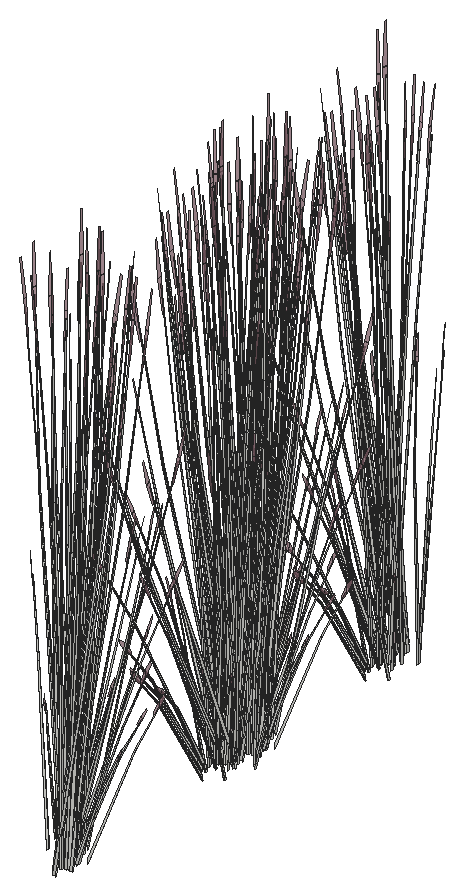
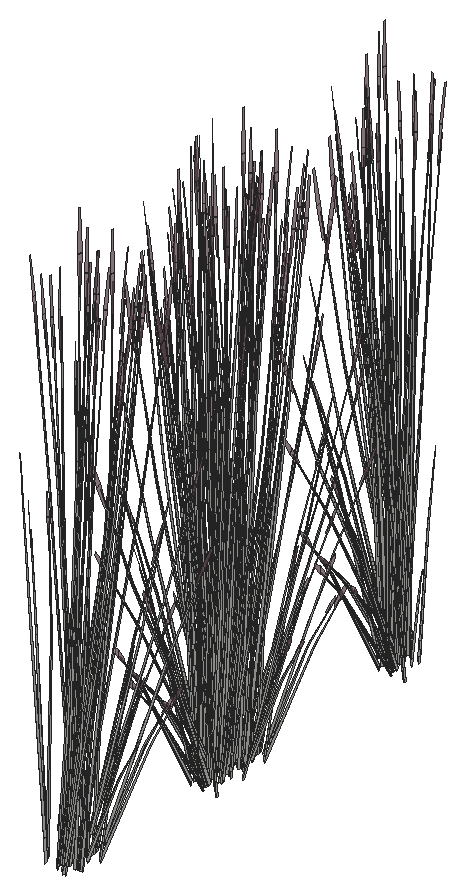
# SketchUp Ruby script. Lengths in inches.
U = 1.inch
M = Sketchup.active_model
def pt(a) = Geom::Point3d.new(a.map { |v| v * U })
def face(e, loops, mat)
  f = e.add_face(loops[0].map { |a| pt(a) })
  loops[1..].each { |l| e.add_face(l.map { |a| pt(a) }).erase! }
  f.material = f.back_material = mat if mat
  f
end
# faces: each face lists its corners as indices into pts; further lists are holes
def faces(e, pts, list, mat = nil) = list.each { |f| face(e, (f[0].is_a?(Array) ? f : [f]).map { |l| l.map { |i| pts[i] } }, mat) }
# xy, xz, yz: faces in a plane at the given z, y or x. An outline is a flat list of corners, or four numbers for a rectangle; further outlines are holes
def ring(l) = l.size == 4 ? [[l[0], l[1]], [l[2], l[1]], [l[2], l[3]], [l[0], l[3]]] : l.each_slice(2).to_a
def flat(e, list, mat, &to3) = list.each { |f| face(e, (f[0].is_a?(Array) ? f : [f]).map { |l| ring(l).map { |u, v| to3.(u, v) } }, mat) }
def xy(e, z, list, mat = nil) = flat(e, list, mat) { |x, y| [x, y, z] }
def xz(e, y, list, mat = nil) = flat(e, list, mat) { |x, z| [x, y, z] }
def yz(e, x, list, mat = nil) = flat(e, list, mat) { |y, z| [x, y, z] }
def lines(e, pts, list) = list.each { |a, b| e.add_line(pt(pts[a]), pt(pts[b])) }
# prism: a flat outline (further loops are holes) pulled along v
def prism(e, loops, v, mat = nil)
  f = face(e, loops, mat); d = Geom::Vector3d.new(v.map { |x| x * U })
  f.pushpull(f.normal.samedirection?(d) ? d.length : -d.length)
end
def box(e, o, s, mat = nil) = prism(e, [[o, [o[0] + s[0], o[1], o[2]], [o[0] + s[0], o[1] + s[1], o[2]], [o[0], o[1] + s[1], o[2]]]], [0, 0, s[2]], mat)
def at(x, y, z, deg = 0) = Geom::Transformation.translation(pt([x, y, z])) * Geom::Transformation.rotation(ORIGIN, Z_AXIS, deg.degrees)
def axes(o, x, y, z) = Geom::Transformation.new([*x, 0, *y, 0, *z, 0, *pt(o).to_a, 1])
def part(name) = M.definitions.add(name)
# library, detail: a bought-in or finely detailed component or shape, given as its bounding box
def library(name, o, s) = part(name).tap { |d| box(d.entities, o, s) }
def detail(e, o, s) = box(e.add_group.entities, o, s)
def put(e, d, t, mat = nil) = e.add_instance(d, t).tap { |i| i.material = mat if mat }
def group(e, t, mat = nil) = e.add_group.tap { |g| g.transformation = t; g.material = mat if mat }.entities
root = M.entities
M.materials.add("LightPink_Translucent").color = [144, 107, 117]
M.materials["LightPink_Translucent"].alpha = 0.75
c1 = part("blade")
p = [[2.15,0.21,22],[0,0.17,0],[0.09,0.45,0],[2.18,0.31,22],[2.29,0.31,22],[0.38,0.45,0],
  [2.48,0.24,33],[2.49,0.24,33],[2.48,0.22,33]]
faces(c1.entities,p,[[0,1,2,3],[4,5,2,3],[6,3,4,7],[8,0,3,6]])
c2 = part("seeds")
p = [[0.3,-0.1,1.38],[-0.01,-0.03,1.59],[-0.01,-0.03,0.03],[0.14,-0.07,-0.07],[0.29,-0.03,3],[0.15,0.01,3.11]]
faces(c2.entities,p,[[0,1,2,3],[1,0,4,5]],"LightPink_Translucent")
c3 = part("blade with seeds")
put(c3.entities,c1,at(0,0,0))
put(c3.entities,c2,axes([2.4,0.25,30.99],[1.5799,-0.05474,1.17369],[-0.12525,1.92788,0.29478],[-0.07173,-0.02425,1.56792]))
put(root,c3,axes([252.5625,62.65,0.99],[-0.2011,-0.44539,0.12804],[0.20266,-0.432,0.25465],[-0.02221,0.09096,1.1642]))
put(root,c3,axes([252.1875,61.98,0.6875],[0.26625,0.10025,-0.45255],[-0.05619,0.61836,-0.11877],[0.07946,0.07493,0.99892]))
put(root,c3,axes([253.36,63.06,1.2],[-0.15814,0.10094,0.83364],[0.07444,-0.41719,0.6125],[0.0839,0.02855,0.18362]))
put(root,c3,axes([251.67,64.27,0.79],[-0.25804,-0.27452,0],[0.12419,-0.5704,0],[0,0,1.1809]))
put(root,c3,axes([251.89,63.54,0.98],[-0.24993,-0.49214,-0.18284],[0.21031,-0.55263,0.40012],[-0.0673,0.05757,1.22088]))
put(root,c3,axes([251.23,64.48,0.99],[0.23955,0.30573,0.36036],[-0.14318,0.54821,0],[-0.05456,-0.06963,1.14313]))
put(root,c3,axes([252.07,62.36,1.17],[0.12419,-0.55096,0.32471],[0.25804,0.26516,-0.15627],[0,0.12701,1.04254]))
put(root,c3,axes([252.03,62.68,0.86],[0,0.70714,-0.04091],[-0.32006,0,0],[0,0.02222,1.30182]))
put(root,c3,axes([252.05,62.18,0.8],[0.15376,0.51322,-0.32471],[-0.2329,0.3614,0.15627],[0.04976,0.0635,1.04254]))
put(root,c3,axes([251.09,64.8,0.91],[-0.16003,0.61271,0],[-0.26773,-0.34169,-0.37456],[-0.06098,-0.07782,1.18819]))
put(root,c3,axes([252.73,62.67,0.99],[0,-0.61145,0.36036],[0.28637,0,0],[0,0.13926,1.14313]))
put(root,c3,axes([252.01,63.13,1.17],[0.27795,-0.03775,0.32471],[0.02514,0.62656,-0.15627],[-0.04976,0.0635,1.04254]))
put(root,c3,axes([252.18,62.49,1.09],[0.23848,-0.17832,0.10509],[0.08351,0.5092,-0.30009],[0,0.11207,0.91989]))
put(root,c3,axes([251.76,63.43,0.8],[-0.27795,0.03775,-0.32471],[-0.02514,-0.62656,0.15627],[-0.04976,0.0635,1.04254]))
put(root,c3,axes([253.07,63.73,1.07],[-0.06164,-0.15038,1.03788],[0.0802,-0.49748,-0.22321],[0.12472,0.06739,0.44375]))
put(root,c3,axes([251.97,64.28,0.79],[0.25804,0.27452,0],[-0.12419,0.5704,0],[0,0,1.26978]))
put(root,c3,axes([252.07,64.88,0.78],[-0.15803,-0.61485,-0.03732],[0.26773,-0.34169,0.37456],[-0.06597,0.05854,1.1876]))
put(root,c3,axes([252.01,63.4,1.09],[0.1891,0.36737,0.10509],[-0.15773,0.41447,-0.30009],[-0.0439,0.05603,0.91989]))
put(root,c3,axes([252.5,64.03,2.81],[0.25586,0.01472,-0.51563],[-0.01718,0.61995,0.06223],[0.1084,0.06542,0.72942]))
put(root,c3,axes([252.21,64.53,0.99],[0.23955,-0.30573,0.36036],[0.14318,0.54821,0],[-0.05456,0.06963,1.14313]))
put(root,c3,axes([251.875,64.05,0.86],[0.11128,0.70245,-0.04364],[-0.31797,0.24614,0],[0.00389,0.02453,1.2496]))
put(root,c3,axes([252,64.81,0.66],[-0.23879,-0.15129,-0.22483],[0.06012,-0.53279,0.22483],[-0.04814,0.06144,1.00865]))
put(root,c3,axes([250.27,63.73,1.07],[0.08895,0.05019,1.03788],[0.05733,0.5127,-0.22321],[-0.12083,0.09597,0.44375]))
put(root,c3,axes([252.92,62.77,0.92],[0.32006,0,0],[0,0.68339,-0.37456],[0,0.15565,1.18819]))
put(root,c3,axes([252.79,63.125,0.79],[-0.3199,-0.00489,-0.03612],[0,-0.68339,0.36248],[-0.01005,0.15557,1.14929]))
put(root,c3,axes([252.1,62.53,1.13],[0.28825,0.29175,-0.21117],[-0.1388,0.61578,-0.36291],[0.00906,0.15119,1.15913]))
put(root,c3,axes([250.09,64.8,1.2],[0.10667,-0.27712,0.83364],[0.04209,0.43871,0.6125],[-0.07709,0.07855,0.18362]))
put(root,c3,axes([252.73,63.22,0.66],[-0.17867,0.3815,-0.22483],[-0.17867,-0.3815,0.22483],[0,0.12288,1.00865]))
put(root,c3,axes([251.96,63.26,1.13],[0.02983,0.6977,-0.21117],[-0.31064,0.04219,-0.36291],[-0.0547,0.09294,1.15913]))
put(root,c3,axes([252.07,62.99,0.8],[-0.12419,0.55096,-0.32471],[-0.25804,-0.26516,0.15627],[0,0.12701,1.04254]))
put(root,c3,axes([251.77,63.79,0.6875],[-0.1724,0.45959,-0.45255],[-0.21416,-0.41674,-0.11877],[-0.06908,0.11465,0.99892]))
put(root,c3,axes([252.08,64.57,0.88],[0.32044,0.19874,0.22322],[-0.08017,0.71038,-0.26485],[-0.05304,0.08891,1.19671]))
put(root,c3,axes([252.05,65.05,0.66],[-0.23955,0.30573,-0.36036],[-0.14318,-0.54821,0],[-0.05456,0.06963,1.14313]))
put(root,c3,axes([252.85,63.24,0.66],[0,0.61145,-0.36036],[-0.28637,0,0],[0,0.13926,1.14313]))
put(root,c3,axes([252.49,64.51,1.2],[-0.14411,-0.17581,0.83364],[0.18609,-0.17864,0.6125],[0.05019,0.15132,0.18362]))
put(root,c3,axes([252.27,64.95,0.91],[0.16003,0.61271,0],[-0.26773,0.34169,-0.37456],[-0.06098,0.07782,1.18819]))
put(root,c3,axes([252.53,65.16,0.28],[0.01865,-0.08828,1.27986],[0.23477,-0.25998,-0.19552],[0.07118,0.13456,0.218]))
put(root,c3,axes([252.13,62.53,1.26],[-0.00699,-0.5757,1.02533],[0.31645,0.14923,0.43413],[-0.07484,0.31502,0.96783]))
put(root,c3,axes([252.22,63.15,0.71],[0.09385,0.55983,-0.50233],[-0.27035,0.20162,-0.13184],[0.01037,0.18957,1.1088]))
put(root,c3,axes([250.37,65.08,0.28],[0.03433,0.06109,1.27986],[0.05822,0.56601,-0.19552],[-0.07609,0.1207,0.218]))
put(root,c3,axes([252.51,65.31,1.13],[-0.16414,-0.01918,0.76251],[0.10839,-0.40729,0.421],[0.06484,0.1447,0.59812]))
put(root,c3,axes([251.97,64.32,1.07],[0.00452,-0.20269,1.03788],[0.21585,-0.22641,-0.22321],[0.06663,0.2426,0.44375]))
put(root,c3,axes([250.99,66.01,1.2],[-0.00662,-0.36357,0.83364],[0.16552,0.25931,0.6125],[-0.03255,0.17329,0.18362]))
put(root,c3,axes([251.43,65.14,0.28],[0.04142,-0.03327,1.27986],[0.24917,0.18313,-0.19552],[0.00729,0.2064,0.218]))
put(root,c3,axes([250.86,65.22,1.24],[0.23252,-0.10828,0.04723],[0.05346,0.43623,-0.62638],[-0.01474,0.22082,0.56147]))
put(root,c3,axes([251.51,64.9,2.81],[0.12216,0.49718,-0.51563],[-0.25147,0.27708,0.06223],[0.02857,0.24022,0.72942]))
put(root,c3,axes([250.8,65.6875,1.07],[0.08077,-0.09646,1.03788],[0.19942,0.29084,-0.22321],[-0.05936,0.25166,0.44375]))
put(root,c3,axes([252.15,78.82,1.07],[-0.07276,0.12376,1.03788],[-0.21789,-0.21662,-0.22321],[0.04039,-0.2694,0.44375]))
put(root,c3,axes([251.82,79.25,2.81],[-0.12216,-0.49718,-0.51563],[0.25147,-0.27708,0.06223],[-0.02857,-0.24022,0.72942]))
put(root,c3,axes([251.03,78.58,1.07],[-0.0155,0.20002,1.03788],[-0.22659,0.16744,-0.22321],[-0.05297,-0.25854,0.44375]))
put(root,c3,axes([251.61,78.14,0.28],[-0.04293,0.02203,1.27986],[-0.23742,-0.24798,-0.19552],[0.00398,-0.20684,0.218]))
put(root,c3,axes([252.33,79.73,2.81],[0.00666,-0.56559,-0.51563],[0.28045,0.03799,0.06223],[0.0296,-0.23961,0.72942]))
put(root,c3,axes([251.88,77.83,1.2],[0.03283,0.35655,0.83364],[-0.18215,-0.19748,0.6125],[0.0196,-0.18257,0.18362]))
put(root,c3,axes([250.95,78.26,1.2],[0.13352,0.21281,0.83364],[-0.19445,0.12793,0.6125],[-0.0416,-0.16355,0.18362]))
put(root,c3,axes([251.27,79.39,2.81],[-0.21825,-0.29555,-0.51563],[0.15511,-0.5179,0.06223],[-0.07907,-0.17646,0.72942]))
put(root,c3,axes([250.84,78.9,0.28],[-0.02479,0.08055,1.27986],[-0.25056,0.17367,-0.19552],[-0.06053,-0.15798,0.218]))
put(root,c3,axes([251.25,81.11,0.72],[-0.10512,-0.62701,-0.50685],[0.30279,-0.22582,-0.13303],[-0.01162,-0.21232,1.11879]))
put(root,c3,axes([252.66,79.2,0.28],[-0.03831,-0.04817,1.27986],[-0.0984,-0.53815,-0.19552],[0.06638,-0.14604,0.218]))
put(root,c3,axes([252.66,80.72,2.81],[0.1337,-0.48245,-0.51563],[0.23429,0.34287,0.06223],[0.07983,-0.1748,0.72942]))
put(root,c3,axes([251.21,79.31,0.91],[-0.16003,-0.61271,0],[0.26773,-0.34169,-0.37456],[0.06098,-0.07782,1.18819]))
put(root,c3,axes([251.56,78.57,0.74],[-0.17688,0.35078,-0.02825],[-0.16207,-0.38418,-0.1281],[-0.01141,-0.10886,0.42251]))
put(root,c3,axes([250.64,81.03,0.66],[0,-0.61145,-0.36036],[0.28637,0,0],[0,-0.13926,1.14313]))
put(root,c3,axes([251.43,79.22,0.66],[0.23955,-0.30573,-0.36036],[0.14318,0.54821,0],[0.05456,-0.06963,1.14313]))
put(root,c3,axes([252.85,80.27,1.07],[-0.09144,-0.01811,1.03788],[-0.09368,-0.48584,-0.22321],[0.11233,-0.13744,0.44375]))
put(root,c3,axes([251.71,80.47,0.6875],[0.1724,-0.45959,-0.45255],[0.21416,0.41674,-0.11877],[0.06908,-0.11465,0.99892]))
put(root,c3,axes([252.96,79.38,1.2],[-0.08525,0.31126,0.83364],[-0.07328,-0.41819,0.6125],[0.07041,-0.10479,0.18362]))
put(root,c3,axes([251.41,81.28,0.8],[0.12419,-0.55096,-0.32471],[0.25804,0.26516,0.15627],[0,-0.12701,1.04254]))
put(root,c3,axes([251.53,81,1.13],[-0.02983,-0.6977,-0.21117],[0.31064,-0.04219,-0.36291],[0.0547,-0.09294,1.15913]))
put(root,c3,axes([250.76,81.04,0.66],[0.17867,-0.3815,-0.22483],[0.17867,0.3815,0.22483],[0,-0.12288,1.00865]))
put(root,c3,axes([250.6875,79.21,0.74],[-0.07384,0.49928,-0.02825],[-0.22725,-0.15358,-0.1281],[-0.0345,-0.08166,0.42251]))
put(root,c3,axes([251.38,81.73,1.13],[-0.28825,-0.29175,-0.21117],[0.1388,-0.61578,-0.36291],[-0.00906,-0.15119,1.15913]))
put(root,c3,axes([250.5625,81.49,0.91],[-0.32006,0,0],[0,-0.68339,-0.37456],[0,-0.15565,1.18819]))
put(root,c3,axes([250.62,80.27,1.07],[0.04997,0.17024,1.03788],[-0.11515,0.46273,-0.22321],[-0.11824,-0.1106,0.44375]))
put(root,c3,axes([251.49,79.46,0.66],[0.23879,0.15129,-0.22483],[-0.06012,0.53279,0.22483],[0.04814,-0.06144,1.00865]))
put(root,c3,axes([250.82,80.12,2.81],[-0.25586,-0.01472,-0.51563],[0.01718,-0.61995,0.06223],[-0.1084,-0.06542,0.72942]))
put(root,c3,axes([250.8125,81.31,0.88],[-0.23808,0.51407,0.22322],[-0.23822,-0.50866,-0.26485],[-0.00831,-0.14599,1.19671]))
put(root,c3,axes([251.57,81.55,0.96],[0.28839,0.29636,0.17466],[-0.1388,0.61578,0.36291],[0,-0.14195,1.16519]))
put(root,c3,axes([251.46,82.38,0.96],[0.06784,-0.72454,-0.17004],[0.32166,0.1263,0.37211],[-0.05621,-0.10006,1.13542]))
put(root,c3,axes([250.32,80.78,1.2],[0.16341,-0.04375,0.83364],[-0.10366,0.38551,0.6125],[-0.08075,-0.05783,0.18362]))
put(root,c3,axes([251.48,81.14,1.17],[-0.27795,0.03775,0.32471],[-0.02514,-0.62656,-0.15627],[0.04976,-0.0635,1.04254]))
put(root,c3,axes([250.76,81.59,0.99],[0,0.61145,0.36036],[-0.28637,0,0],[0,-0.13926,1.14313]))
put(root,c3,axes([252.39,79.46,0.92],[0.16003,-0.61271,0],[0.26773,0.34169,-0.37456],[0.06098,0.07782,1.18819]))
put(root,c3,axes([251.43,82.09,0.8],[-0.15376,-0.51322,-0.32471],[0.2329,-0.3614,0.15627],[-0.04976,-0.0635,1.04254]))
put(root,c3,axes([251.47,81.36,0.91],[0.11128,0.68373,0.33208],[-0.31797,0.23776,0.13031],[0.00389,-0.12563,1.15295]))
put(root,c3,axes([253.02,81.89,0.63],[-0.16485,0.07338,1.02759],[-0.02624,-0.58408,0.05882],[0.11546,-0.08841,0.58473]))
put(root,c3,axes([253.32,81.37,0.83],[-0.15869,-0.39099,-0.04709],[0.1738,-0.35825,-0.21349],[0.04925,-0.02522,0.70419]))
put(root,c3,axes([251.41,81.9,1.17],[-0.12419,0.55096,0.32471],[-0.25804,-0.26516,-0.15627],[0,-0.12701,1.04254]))
put(root,c3,axes([251.87,81.42,0.79],[0,-0.70749,0],[0.32006,0,0],[0,0,1.30246]))
put(root,c3,axes([252.25,79.78,0.99],[-0.23955,-0.30573,0.36036],[0.14318,-0.54821,0],[0.05456,0.06963,1.14313]))
put(root,c3,axes([252.72,81.93,2.81],[0.22491,-0.27005,-0.51563],[0.12534,0.55588,0.06223],[0.10867,-0.06315,0.72942]))
put(root,c3,axes([251.3,82.28,0.6875],[-0.26625,-0.10025,-0.45255],[0.05619,-0.61836,-0.11877],[-0.07946,-0.07493,0.99892]))
put(root,c3,axes([251.71,80.97,0.91],[-0.21222,0.5549,0.33208],[-0.25213,-0.48983,0.13031],[0.05116,-0.05538,1.15295]))
put(root,c3,axes([251.95,81.97,0.86],[-0.23808,-0.52628,-0.0445],[0.23822,-0.5266,0],[-0.00831,-0.01838,1.27426]))
put(root,c3,axes([251.35,80.06,0.99],[-0.07394,0.60768,0.12804],[-0.27057,-0.17197,0.25465],[0.04674,-0.00296,1.1642]))
put(root,c3,axes([251.23,80.55,0.35],[-0.25194,0.2448,0.93574],[-0.08019,-0.7024,0.36359],[0.1547,0.01169,1.0643]))
put(root,c3,axes([251.91,80.74,1.09],[0.04938,-0.54569,0.10509],[0.24125,0.09472,-0.30009],[0.0439,0.05603,0.91989]))
put(root,c3,axes([251.49,82.03,0.91],[0.32351,0.12883,0.33208],[-0.06584,0.72759,0.13031],[-0.04728,-0.07026,1.15295]))
put(root,c3,axes([253.2,81.5,0.28],[-0.01338,-0.09283,1.27986],[0.09278,-0.54301,-0.19552],[0.09359,-0.00781,0.218]))
put(root,c3,axes([250.44,81.41,0.28],[0.00649,0.09636,1.27986],[-0.13086,0.50324,-0.19552],[-0.09295,-0.02537,0.218]))
put(root,c3,axes([251.81,80.88,1.17],[-0.15376,-0.51322,0.32471],[0.2329,-0.3614,-0.15627],[0.04976,0.0635,1.04254]))
put(root,c3,axes([251.01,83.23,0.66],[-0.06012,-0.53279,-0.22483],[0.23879,-0.15129,0.22483],[-0.04814,-0.06144,1.00865]))
put(root,c3,axes([251.32,83.19,0.99],[0.27504,-0.16229,0.12804],[0.06792,0.60396,0.25465],[-0.02453,-0.088,1.1642]))
put(root,c3,axes([251.89,80.91,1.13],[0.25843,-0.40595,-0.21117],[0.17185,0.5736,-0.36291],[0.06376,0.05825,1.15913]))
put(root,c3,axes([250.95,83.45,0.66],[-0.23955,-0.30573,-0.36036],[0.14318,-0.54821,0],[-0.05456,-0.06963,1.14313]))
put(root,c3,axes([252.54,79.83,0.66],[0.23955,0.30573,-0.36036],[-0.14318,0.54821,0],[0.05456,0.06963,1.14313]))
put(root,c3,axes([252.08,81.58,0.79],[0.28637,0,0],[0,0.63302,0],[0,0,1.29484]))
put(root,c3,axes([251.6,82.375,1.13],[-0.25843,0.40595,-0.21117],[-0.17185,-0.5736,-0.36291],[-0.06376,-0.05825,1.15913]))
put(root,c3,axes([252.16,80.09,0.99],[-0.27504,0.16229,0.12804],[-0.06792,-0.60396,0.25465],[0.02453,0.088,1.1642]))
put(root,c3,axes([252.47,80.0625,0.66],[0.06012,0.53279,-0.22483],[-0.23879,0.15129,0.22483],[0.04814,0.06144,1.00865]))
put(root,c3,axes([251.99,81.26,0.92],[-0.32351,-0.12883,0.35707],[0.06584,-0.72759,0.14012],[0.04728,0.07026,1.23973]))
put(root,c3,axes([251.73,83.05,0.79],[-0.08351,-0.52716,0],[0.23848,-0.18461,0],[0,0,1.1204]))
put(root,c3,axes([251.57,82.55,1.09],[-0.04938,0.54569,0.10509],[-0.24125,-0.09472,-0.30009],[-0.0439,-0.05603,0.91989]))
put(root,c3,axes([252.05,82.98,0.78],[0.26872,-0.20746,-0.13933],[0.09442,0.59762,0.00006],[0.02966,-0.02293,1.26212]))
put(root,c3,axes([252.14,83.23,0.99],[0.07394,-0.60768,0.12804],[0.27057,0.17197,0.25465],[-0.04674,0.00296,1.1642]))
put(root,c3,axes([252.08,81.85,0.8],[0.17867,0.39495,0],[-0.17867,0.39495,0],[0,0,1.22851]))
put(root,c3,axes([252.5625,81.68,0.99],[-0.2011,-0.44539,0.12804],[0.20266,-0.432,0.25465],[-0.02221,0.09096,1.1642]))
put(root,c3,axes([252.1875,81,0.6875],[0.26625,0.10025,-0.45255],[-0.05619,0.61836,-0.11877],[0.07946,0.07493,0.99892]))
put(root,c3,axes([253.36,82.08,1.2],[-0.15814,0.10094,0.83364],[0.07444,-0.41719,0.6125],[0.0839,0.02855,0.18362]))
put(root,c3,axes([251.67,83.29,0.79],[-0.25804,-0.27452,0],[0.12419,-0.5704,0],[0,0,1.1809]))
put(root,c3,axes([251.89,82.56,0.98],[-0.24993,-0.49214,-0.18284],[0.21031,-0.55263,0.40012],[-0.0673,0.05757,1.22088]))
put(root,c3,axes([251.23,83.5,0.99],[0.23955,0.30573,0.36036],[-0.14318,0.54821,0],[-0.05456,-0.06963,1.14313]))
put(root,c3,axes([252.07,81.39,1.17],[0.12419,-0.55096,0.32471],[0.25804,0.26516,-0.15627],[0,0.12701,1.04254]))
put(root,c3,axes([252.03,81.7,0.86],[0,0.70714,-0.04091],[-0.32006,0,0],[0,0.02222,1.30182]))
put(root,c3,axes([252.05,81.2,0.8],[0.15376,0.51322,-0.32471],[-0.2329,0.3614,0.15627],[0.04976,0.0635,1.04254]))
put(root,c3,axes([251.09,83.82,0.91],[-0.16003,0.61271,0],[-0.26773,-0.34169,-0.37456],[-0.06098,-0.07782,1.18819]))
put(root,c3,axes([252.73,81.69,0.99],[0,-0.61145,0.36036],[0.28637,0,0],[0,0.13926,1.14313]))
put(root,c3,axes([252.01,82.15,1.17],[0.27795,-0.03775,0.32471],[0.02514,0.62656,-0.15627],[-0.04976,0.0635,1.04254]))
put(root,c3,axes([252.18,81.51,1.09],[0.23848,-0.17832,0.10509],[0.08351,0.5092,-0.30009],[0,0.11207,0.91989]))
put(root,c3,axes([251.76,82.46,0.8],[-0.27795,0.03775,-0.32471],[-0.02514,-0.62656,0.15627],[-0.04976,0.0635,1.04254]))
put(root,c3,axes([253.07,82.75,1.07],[-0.06164,-0.15038,1.03788],[0.0802,-0.49748,-0.22321],[0.12472,0.06739,0.44375]))
put(root,c3,axes([251.97,83.3,0.79],[0.25804,0.27452,0],[-0.12419,0.5704,0],[0,0,1.26978]))
put(root,c3,axes([252.07,83.91,0.78],[-0.15803,-0.61485,-0.03732],[0.26773,-0.34169,0.37456],[-0.06597,0.05854,1.1876]))
put(root,c3,axes([252.01,82.42,1.09],[0.1891,0.36737,0.10509],[-0.15773,0.41447,-0.30009],[-0.0439,0.05603,0.91989]))
put(root,c3,axes([252.5,83.06,2.81],[0.25586,0.01472,-0.51563],[-0.01718,0.61995,0.06223],[0.1084,0.06542,0.72942]))
put(root,c3,axes([252.21,83.55,0.99],[0.23955,-0.30573,0.36036],[0.14318,0.54821,0],[-0.05456,0.06963,1.14313]))
put(root,c3,axes([251.875,83.07,0.86],[0.11128,0.70245,-0.04364],[-0.31797,0.24614,0],[0.00389,0.02453,1.2496]))
put(root,c3,axes([252,83.83,0.66],[-0.23879,-0.15129,-0.22483],[0.06012,-0.53279,0.22483],[-0.04814,0.06144,1.00865]))
put(root,c3,axes([250.27,82.75,1.07],[0.08895,0.05019,1.03788],[0.05733,0.5127,-0.22321],[-0.12083,0.09597,0.44375]))
put(root,c3,axes([252.92,81.8,0.92],[0.32006,0,0],[0,0.68339,-0.37456],[0,0.15565,1.18819]))
put(root,c3,axes([252.79,82.15,0.79],[-0.3199,-0.00489,-0.03612],[0,-0.68339,0.36248],[-0.01005,0.15557,1.14929]))
put(root,c3,axes([252.1,81.55,1.13],[0.28825,0.29175,-0.21117],[-0.1388,0.61578,-0.36291],[0.00906,0.15119,1.15913]))
put(root,c3,axes([250.09,83.82,1.2],[0.10667,-0.27712,0.83364],[0.04209,0.43871,0.6125],[-0.07709,0.07855,0.18362]))
put(root,c3,axes([252.73,82.25,0.66],[-0.17867,0.3815,-0.22483],[-0.17867,-0.3815,0.22483],[0,0.12288,1.00865]))
put(root,c3,axes([251.96,82.29,1.13],[0.02983,0.6977,-0.21117],[-0.31064,0.04219,-0.36291],[-0.0547,0.09294,1.15913]))
put(root,c3,axes([252.07,82.01,0.8],[-0.12419,0.55096,-0.32471],[-0.25804,-0.26516,0.15627],[0,0.12701,1.04254]))
put(root,c3,axes([251.77,82.82,0.6875],[-0.1724,0.45959,-0.45255],[-0.21416,-0.41674,-0.11877],[-0.06908,0.11465,0.99892]))
put(root,c3,axes([252.08,83.59,0.88],[0.32044,0.19874,0.22322],[-0.08017,0.71038,-0.26485],[-0.05304,0.08891,1.19671]))
put(root,c3,axes([252.05,84.07,0.66],[-0.23955,0.30573,-0.36036],[-0.14318,-0.54821,0],[-0.05456,0.06963,1.14313]))
put(root,c3,axes([252.85,82.26,0.66],[0,0.61145,-0.36036],[-0.28637,0,0],[0,0.13926,1.14313]))
put(root,c3,axes([252.49,83.53,1.2],[-0.14411,-0.17581,0.83364],[0.18609,-0.17864,0.6125],[0.05019,0.15132,0.18362]))
put(root,c3,axes([252.27,83.98,0.91],[0.16003,0.61271,0],[-0.26773,0.34169,-0.37456],[-0.06098,0.07782,1.18819]))
put(root,c3,axes([252.53,84.18,0.28],[0.01865,-0.08828,1.27986],[0.23477,-0.25998,-0.19552],[0.07118,0.13456,0.218]))
put(root,c3,axes([252.13,81.55,1.26],[-0.00699,-0.5757,1.02533],[0.31645,0.14923,0.43413],[-0.07484,0.31502,0.96783]))
put(root,c3,axes([252.22,82.18,0.71],[0.09385,0.55983,-0.50233],[-0.27035,0.20162,-0.13184],[0.01037,0.18957,1.1088]))
put(root,c3,axes([250.37,84.11,0.28],[0.03433,0.06109,1.27986],[0.05822,0.56601,-0.19552],[-0.07609,0.1207,0.218]))
put(root,c3,axes([252.51,84.33,1.13],[-0.16414,-0.01918,0.76251],[0.10839,-0.40729,0.421],[0.06484,0.1447,0.59812]))
put(root,c3,axes([251.97,83.34,1.07],[0.00452,-0.20269,1.03788],[0.21585,-0.22641,-0.22321],[0.06663,0.2426,0.44375]))
put(root,c3,axes([250.99,85.03,1.2],[-0.00662,-0.36357,0.83364],[0.16552,0.25931,0.6125],[-0.03255,0.17329,0.18362]))
put(root,c3,axes([251.43,84.16,0.28],[0.04142,-0.03327,1.27986],[0.24917,0.18313,-0.19552],[0.00729,0.2064,0.218]))
put(root,c3,axes([250.86,84.25,1.24],[0.23252,-0.10828,0.04723],[0.05346,0.43623,-0.62638],[-0.01474,0.22082,0.56147]))
put(root,c3,axes([251.51,83.93,2.81],[0.12216,0.49718,-0.51563],[-0.25147,0.27708,0.06223],[0.02857,0.24022,0.72942]))
put(root,c3,axes([250.8,84.71,1.07],[0.08077,-0.09646,1.03788],[0.19942,0.29084,-0.22321],[-0.05936,0.25166,0.44375]))
put(root,c3,axes([252.15,95.39,1.07],[-0.07276,0.12376,1.03788],[-0.21789,-0.21662,-0.22321],[0.04039,-0.2694,0.44375]))
put(root,c3,axes([251.03,95.16,1.07],[-0.0155,0.20002,1.03788],[-0.22659,0.16744,-0.22321],[-0.05297,-0.25854,0.44375]))
put(root,c3,axes([251.61,94.72,0.28],[-0.04293,0.02203,1.27986],[-0.23742,-0.24798,-0.19552],[0.00398,-0.20684,0.218]))
put(root,c3,axes([251.88,94.41,1.2],[0.03283,0.35655,0.83364],[-0.18215,-0.19748,0.6125],[0.0196,-0.18257,0.18362]))
put(root,c3,axes([250.95,94.84,1.2],[0.13352,0.21281,0.83364],[-0.19445,0.12793,0.6125],[-0.0416,-0.16355,0.18362]))
put(root,c3,axes([251.27,95.96,2.81],[-0.21825,-0.29555,-0.51563],[0.15511,-0.5179,0.06223],[-0.07907,-0.17646,0.72942]))
put(root,c3,axes([250.84,95.48,0.28],[-0.02479,0.08055,1.27986],[-0.25056,0.17367,-0.19552],[-0.06053,-0.15798,0.218]))
put(root,c3,axes([251.25,97.69,0.72],[-0.10512,-0.62701,-0.50685],[0.30279,-0.22582,-0.13303],[-0.01162,-0.21232,1.11879]))
put(root,c3,axes([252.66,95.77,0.28],[-0.03831,-0.04817,1.27986],[-0.0984,-0.53815,-0.19552],[0.06638,-0.14604,0.218]))
put(root,c3,axes([252.66,97.29,2.81],[0.1337,-0.48245,-0.51563],[0.23429,0.34287,0.06223],[0.07983,-0.1748,0.72942]))
put(root,c3,axes([251.21,95.89,0.91],[-0.16003,-0.61271,0],[0.26773,-0.34169,-0.37456],[0.06098,-0.07782,1.18819]))
put(root,c3,axes([251.56,95.15,0.74],[-0.17688,0.35078,-0.02825],[-0.16207,-0.38418,-0.1281],[-0.01141,-0.10886,0.42251]))
put(root,c3,axes([250.64,97.6,0.66],[0,-0.61145,-0.36036],[0.28637,0,0],[0,-0.13926,1.14313]))
put(root,c3,axes([251.43,95.79,0.66],[0.23955,-0.30573,-0.36036],[0.14318,0.54821,0],[0.05456,-0.06963,1.14313]))
put(root,c3,axes([252.85,96.85,1.07],[-0.09144,-0.01811,1.03788],[-0.09368,-0.48584,-0.22321],[0.11233,-0.13744,0.44375]))
put(root,c3,axes([251.71,97.05,0.6875],[0.1724,-0.45959,-0.45255],[0.21416,0.41674,-0.11877],[0.06908,-0.11465,0.99892]))
put(root,c3,axes([252.96,95.96,1.2],[-0.08525,0.31126,0.83364],[-0.07328,-0.41819,0.6125],[0.07041,-0.10479,0.18362]))
put(root,c3,axes([251.41,97.85,0.8],[0.12419,-0.55096,-0.32471],[0.25804,0.26516,0.15627],[0,-0.12701,1.04254]))
put(root,c3,axes([251.53,97.58,1.13],[-0.02983,-0.6977,-0.21117],[0.31064,-0.04219,-0.36291],[0.0547,-0.09294,1.15913]))
put(root,c3,axes([250.76,97.62,0.66],[0.17867,-0.3815,-0.22483],[0.17867,0.3815,0.22483],[0,-0.12288,1.00865]))
put(root,c3,axes([250.6875,95.79,0.74],[-0.07384,0.49928,-0.02825],[-0.22725,-0.15358,-0.1281],[-0.0345,-0.08166,0.42251]))
put(root,c3,axes([251.38,98.3125,1.13],[-0.28825,-0.29175,-0.21117],[0.1388,-0.61578,-0.36291],[-0.00906,-0.15119,1.15913]))
put(root,c3,axes([250.5625,98.07,0.91],[-0.32006,0,0],[0,-0.68339,-0.37456],[0,-0.15565,1.18819]))
put(root,c3,axes([250.62,96.85,1.07],[0.04997,0.17024,1.03788],[-0.11515,0.46273,-0.22321],[-0.11824,-0.1106,0.44375]))
put(root,c3,axes([251.49,96.03,0.66],[0.23879,0.15129,-0.22483],[-0.06012,0.53279,0.22483],[0.04814,-0.06144,1.00865]))
put(root,c3,axes([250.82,96.69,2.81],[-0.25586,-0.01472,-0.51563],[0.01718,-0.61995,0.06223],[-0.1084,-0.06542,0.72942]))
put(root,c3,axes([250.8125,97.89,0.88],[-0.23808,0.51407,0.22322],[-0.23822,-0.50866,-0.26485],[-0.00831,-0.14599,1.19671]))
put(root,c3,axes([251.57,98.125,0.96],[0.28839,0.29636,0.17466],[-0.1388,0.61578,0.36291],[0,-0.14195,1.16519]))
put(root,c3,axes([251.46,98.96,0.96],[0.06784,-0.72454,-0.17004],[0.32166,0.1263,0.37211],[-0.05621,-0.10006,1.13542]))
put(root,c3,axes([250.32,97.36,1.2],[0.16341,-0.04375,0.83364],[-0.10366,0.38551,0.6125],[-0.08075,-0.05783,0.18362]))
put(root,c3,axes([251.48,97.71,1.17],[-0.27795,0.03775,0.32471],[-0.02514,-0.62656,-0.15627],[0.04976,-0.0635,1.04254]))
put(root,c3,axes([250.76,98.17,0.99],[0,0.61145,0.36036],[-0.28637,0,0],[0,-0.13926,1.14313]))
put(root,c3,axes([252.39,96.04,0.92],[0.16003,-0.61271,0],[0.26773,0.34169,-0.37456],[0.06098,0.07782,1.18819]))
put(root,c3,axes([251.43,98.66,0.8],[-0.15376,-0.51322,-0.32471],[0.2329,-0.3614,0.15627],[-0.04976,-0.0635,1.04254]))
put(root,c3,axes([251.47,97.94,0.91],[0.11128,0.68373,0.33208],[-0.31797,0.23776,0.13031],[0.00389,-0.12563,1.15295]))
put(root,c3,axes([253.02,98.46,0.63],[-0.16485,0.07338,1.02759],[-0.02624,-0.58408,0.05882],[0.11546,-0.08841,0.58473]))
put(root,c3,axes([253.32,97.95,0.83],[-0.15869,-0.39099,-0.04709],[0.1738,-0.35825,-0.21349],[0.04925,-0.02522,0.70419]))
put(root,c3,axes([251.41,98.48,1.17],[-0.12419,0.55096,0.32471],[-0.25804,-0.26516,-0.15627],[0,-0.12701,1.04254]))
put(root,c3,axes([251.87,98,0.79],[0,-0.70749,0],[0.32006,0,0],[0,0,1.30246]))
put(root,c3,axes([252.25,96.36,0.99],[-0.23955,-0.30573,0.36036],[0.14318,-0.54821,0],[0.05456,0.06963,1.14313]))
put(root,c3,axes([252.72,98.51,2.81],[0.22491,-0.27005,-0.51563],[0.12534,0.55588,0.06223],[0.10867,-0.06315,0.72942]))
put(root,c3,axes([251.3,98.86,0.6875],[-0.26625,-0.10025,-0.45255],[0.05619,-0.61836,-0.11877],[-0.07946,-0.07493,0.99892]))
put(root,c3,axes([251.71,97.55,0.91],[-0.21222,0.5549,0.33208],[-0.25213,-0.48983,0.13031],[0.05116,-0.05538,1.15295]))
put(root,c3,axes([251.95,98.55,0.86],[-0.23808,-0.52628,-0.0445],[0.23822,-0.5266,0],[-0.00831,-0.01838,1.27426]))
put(root,c3,axes([251.35,96.64,0.99],[-0.07394,0.60768,0.12804],[-0.27057,-0.17197,0.25465],[0.04674,-0.00296,1.1642]))
